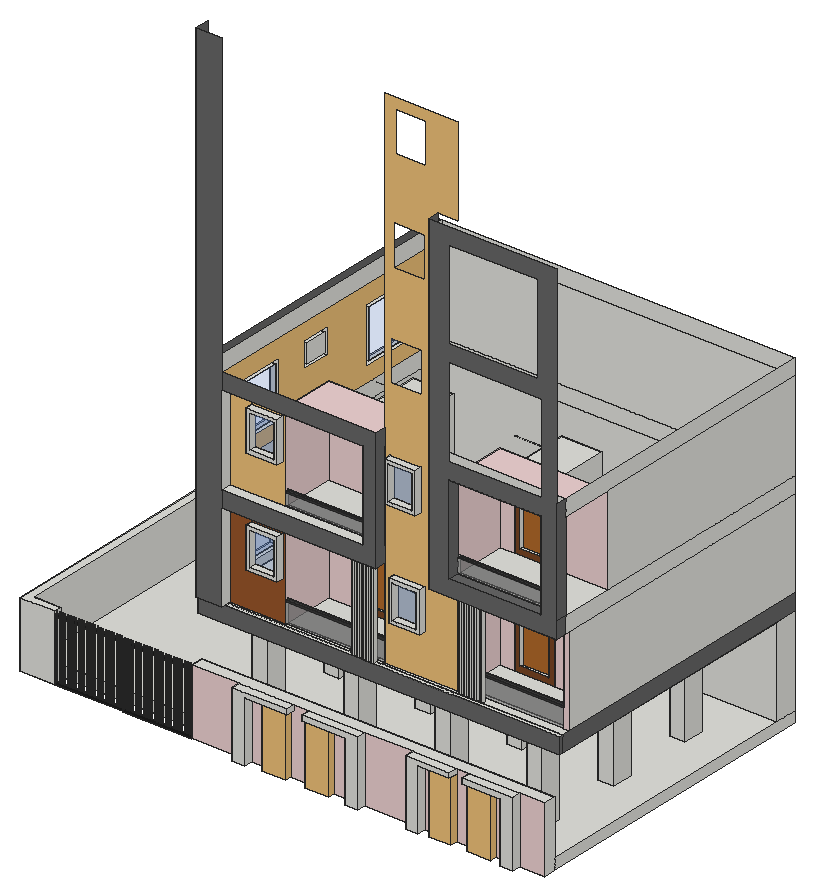
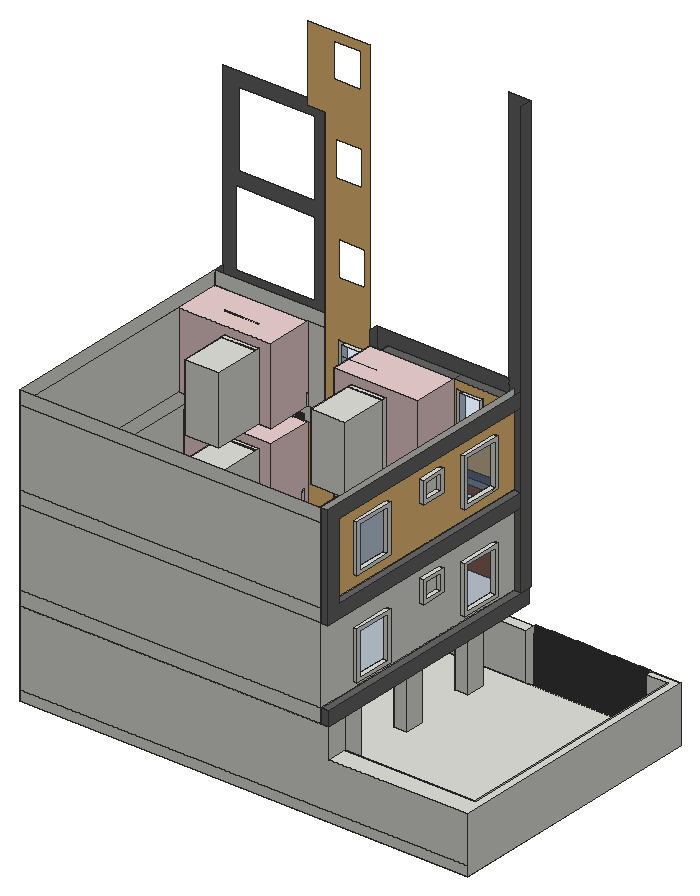
# SketchUp Ruby script. Lengths in inches.
U = 1.inch
M = Sketchup.active_model
def pt(a) = Geom::Point3d.new(a.map { |v| v * U })
def face(e, loops, mat)
  f = e.add_face(loops[0].map { |a| pt(a) })
  loops[1..].each { |l| e.add_face(l.map { |a| pt(a) }).erase! }
  f.material = f.back_material = mat if mat
  f
end
# faces: each face lists its corners as indices into pts; further lists are holes
def faces(e, pts, list, mat = nil) = list.each { |f| face(e, (f[0].is_a?(Array) ? f : [f]).map { |l| l.map { |i| pts[i] } }, mat) }
# xy, xz, yz: faces in a plane at the given z, y or x. An outline is a flat list of corners, or four numbers for a rectangle; further outlines are holes
def ring(l) = l.size == 4 ? [[l[0], l[1]], [l[2], l[1]], [l[2], l[3]], [l[0], l[3]]] : l.each_slice(2).to_a
def flat(e, list, mat, &to3) = list.each { |f| face(e, (f[0].is_a?(Array) ? f : [f]).map { |l| ring(l).map { |u, v| to3.(u, v) } }, mat) }
def xy(e, z, list, mat = nil) = flat(e, list, mat) { |x, y| [x, y, z] }
def xz(e, y, list, mat = nil) = flat(e, list, mat) { |x, z| [x, y, z] }
def yz(e, x, list, mat = nil) = flat(e, list, mat) { |y, z| [x, y, z] }
def lines(e, pts, list) = list.each { |a, b| e.add_line(pt(pts[a]), pt(pts[b])) }
# prism: a flat outline (further loops are holes) pulled along v
def prism(e, loops, v, mat = nil)
  f = face(e, loops, mat); d = Geom::Vector3d.new(v.map { |x| x * U })
  f.pushpull(f.normal.samedirection?(d) ? d.length : -d.length)
end
def box(e, o, s, mat = nil) = prism(e, [[o, [o[0] + s[0], o[1], o[2]], [o[0] + s[0], o[1] + s[1], o[2]], [o[0], o[1] + s[1], o[2]]]], [0, 0, s[2]], mat)
def at(x, y, z, deg = 0) = Geom::Transformation.translation(pt([x, y, z])) * Geom::Transformation.rotation(ORIGIN, Z_AXIS, deg.degrees)
def axes(o, x, y, z) = Geom::Transformation.new([*x, 0, *y, 0, *z, 0, *pt(o).to_a, 1])
def part(name) = M.definitions.add(name)
# library, detail: a bought-in or finely detailed component or shape, given as its bounding box
def library(name, o, s) = part(name).tap { |d| box(d.entities, o, s) }
def detail(e, o, s) = box(e.add_group.entities, o, s)
def put(e, d, t, mat = nil) = e.add_instance(d, t).tap { |i| i.material = mat if mat }
def group(e, t, mat = nil) = e.add_group.tap { |g| g.transformation = t; g.material = mat if mat }.entities
root = M.entities
M.materials.add("Generic").color = [103, 103, 103]
M.materials.add("Generic\#1").color = [239, 210, 210]
M.materials.add("[Color M07]").color = [58, 58, 58]
M.materials.add("[Color M08]").color = [30, 30, 30]
M.materials.add("[Translucent Glass Blue]").color = [98, 147, 234]
M.materials["[Translucent Glass Blue]"].alpha = 0.25
M.materials.add("[Translucent Glass Gray]").color = [128, 128, 128]
M.materials["[Translucent Glass Gray]"].alpha = 0.5
M.materials.add("[Wood Bamboo]").color = [177, 105, 43]
M.materials.add("[Wood Cherry Original]").color = [152, 86, 42]
M.materials.add("[Wood OSB]").color = [240, 195, 122]
M.materials.add("[Wood Veneer 01]").color = [120, 70, 37]
c1 = part("Group\#428")
prism(c1.entities,[[[0,1.97,0],[0,1.97,1.18],[0,0,1.18],[0,0,0]],[[0,1.92,1.13],[0,1.92,0.05],[0,0.05,0.05],[0,0.05,1.13]]],[98.43,0,0])
c2 = part("Group\#430")
xy(c2.entities,0,[[0.3,0,0.22,0.01,0.15,0.04,0.09,0.09,0.04,0.15,0.01,0.22,0,0.3,0.3,0.3],[0.3,0,0.3,0.3,0.59,0.3,0.58,0.22,0.55,0.15,0.5,0.09,0.44,0.04,0.37,0.01],[0,0.3,0.01,0.37,0.04,0.44,0.09,0.5,0.15,0.55,0.22,0.58,0.3,0.59,0.3,0.3],[0.3,0.3,0.3,0.59,0.37,0.58,0.44,0.55,0.5,0.5,0.55,0.44,0.58,0.37,0.59,0.3]])
xy(c2.entities,39.37,[[0.3,0,0.37,0.01,0.44,0.04,0.5,0.09,0.55,0.15,0.58,0.22,0.59,0.3,0.58,0.37,0.55,0.44,0.5,0.5,0.44,0.55,0.37,0.58,0.3,0.59,0.22,0.58,0.15,0.55,0.09,0.5,0.04,0.44,0.01,0.37,0,0.3,0.01,0.22,0.04,0.15,0.09,0.09,0.15,0.04,0.22,0.01]])
p = [[0.09,0.09,0],[0.15,0.04,0],[0.15,0.04,39.37],[0.09,0.09,39.37],[0.22,0.01,0],[0.22,0.01,39.37],
  [0.3,0,0],[0.3,0,39.37],[0.37,0.01,0],[0.37,0.01,39.37],[0.44,0.04,0],[0.44,0.04,39.37],
  [0.5,0.09,0],[0.5,0.09,39.37],[0.01,0.22,0],[0.04,0.15,0],[0.04,0.15,39.37],[0.01,0.22,39.37],
  [0.55,0.15,0],[0.55,0.15,39.37],[0.58,0.22,0],[0.58,0.22,39.37],[0,0.3,0],[0,0.3,39.37],
  [0.59,0.3,0],[0.59,0.3,39.37],[0.01,0.37,0],[0.01,0.37,39.37],[0.58,0.37,0],[0.58,0.37,39.37],
  [0.09,0.5,0],[0.04,0.44,0],[0.04,0.44,39.37],[0.09,0.5,39.37],[0.55,0.44,0],[0.5,0.5,0],
  [0.5,0.5,39.37],[0.55,0.44,39.37],[0.15,0.55,0],[0.15,0.55,39.37],[0.44,0.55,0],[0.44,0.55,39.37],
  [0.22,0.58,0],[0.22,0.58,39.37],[0.3,0.59,0],[0.3,0.59,39.37],[0.37,0.58,0],[0.37,0.58,39.37]]
faces(c2.entities,p,[[0,1,2,3],[1,4,5,2],[4,6,7,5],[6,8,9,7],[8,10,11,9],[10,12,13,11],[14,15,16,17],[15,0,3,16],
  [12,18,19,13],[18,20,21,19],[22,14,17,23],[20,24,25,21],[26,22,23,27],[24,28,29,25],[30,31,32,33],[31,26,27,32],
  [34,35,36,37],[28,34,37,29],[38,30,33,39],[35,40,41,36],[42,38,39,43],[44,42,43,45],[46,44,45,47],[40,46,47,41]])
c3 = part("Group\#429")
prism(c3.entities,[[[0.01,0.22,35.83],[0,0.3,35.83],[0.01,0.37,35.83],[0.04,0.44,35.83],[0.09,0.5,35.83],[0.15,0.55,35.83],[0.22,0.58,35.83],[0.3,0.59,35.83],[0.37,0.58,35.83],[0.44,0.55,35.83],[0.5,0.5,35.83],[0.55,0.44,35.83],[0.58,0.37,35.83],[0.59,0.3,35.83],[0.58,0.22,35.83],[0.55,0.15,35.83],[0.5,0.09,35.83],[0.44,0.04,35.83],[0.37,0.01,35.83],[0.3,0,35.83],[0.22,0.01,35.83],[0.15,0.04,35.83],[0.09,0.09,35.83],[0.04,0.15,35.83]]],[0,0,3.54])
c4 = part("Barred gate panel")
g1 = group(c4.entities,at(0,0,0))
put(g1,c1,axes([0,0,39.76],[1,0,0],[0,0,-1],[0,1,0]),"[Color M08]")
put(g1,c1,axes([0,0,1.97],[1,0,0],[0,0,-1],[0,1,0]),"[Color M08]")
put(g1,c1,axes([98.43,0,37.8],[0,0,-0.364],[-1,0,0],[0,1,0]),"[Color M08]")
put(g1,c1,axes([1.97,0,37.8],[0,0,-0.364],[-1,0,0],[0,1,0]),"[Color M08]")
g2 = group(c4.entities,at(1.67,0.3,1.97))
put(g2,c2,at(78.74,0,0),"[Color M08]")
put(g2,c2,at(90.55,0,0),"[Color M08]")
put(g2,c2,at(82.68,0,0),"[Color M08]")
put(g2,c2,at(86.61,0,0),"[Color M08]")
put(g2,c2,at(66.93,0,0),"[Color M08]")
put(g2,c2,at(11.8125,0,0),"[Color M08]")
put(g2,c2,at(15.75,0,0),"[Color M08]")
put(g2,c2,at(47.24,0,0),"[Color M08]")
put(g2,c2,at(59.06,0,0),"[Color M08]")
put(g2,c3,at(0,0,0),"[Color M08]")
put(g2,c2,at(39.37,0,0),"[Color M08]")
put(g2,c2,at(62.99,0,0),"[Color M08]")
put(g2,c2,at(55.12,0,0),"[Color M08]")
put(g2,c2,at(19.69,0,0),"[Color M08]")
put(g2,c2,at(35.43,0,0),"[Color M08]")
put(g2,c2,at(7.875,0,0),"[Color M08]")
put(g2,c2,at(23.62,0,0),"[Color M08]")
put(g2,c2,at(31.5,0,0),"[Color M08]")
put(g2,c2,at(43.31,0,0),"[Color M08]")
put(g2,c2,at(27.56,0,0),"[Color M08]")
put(g2,c2,at(3.9375,0,0),"[Color M08]")
put(g2,c2,at(51.18,0,0),"[Color M08]")
put(g2,c2,at(70.87,0,0),"[Color M08]")
put(g2,c2,at(74.8,0,0),"[Color M08]")
put(g2,c3,at(94.49,0,0),"[Color M08]")
c5 = part("Group\#1")
xy(c5.entities,0,[[0,0,76.25,8.9375]])
xy(c5.entities,11.01,[[11.01,0,65.24,5.9375]])
xy(c5.entities,138.8,[[11.01,0,65.24,5.9375]])
xy(c5.entities,149.8125,[[0,0,76.25,8.9375]])
xz(c5.entities,0,[[[0,0,76.25,149.8125],[11.01,11.01,65.24,138.8]]],"[Wood Veneer 01]")
xz(c5.entities,5.9375,[[11.01,11.01,65.24,138.8]],"[Wood Bamboo]")
xz(c5.entities,8.9375,[[0,0,76.25,149.8125]])
yz(c5.entities,0,[[0,0,8.9375,149.8125]])
yz(c5.entities,11.01,[[0,11.01,5.9375,138.8]])
yz(c5.entities,65.24,[[0,11.01,5.9375,138.8]])
yz(c5.entities,76.25,[[0,0,8.9375,149.8125]])
xy(root,-20.9375,[[412.81,0,412.81,16.75,323.875,16.75,323.875,40.1875,989.0625,40.1875,989.0625,16.75,942.13,16.75,942.13,0,918.69,0,918.69,16.75,897.59,16.75,897.59,4.0625,852.34,4.0625,852.34,16.75,822.94,16.75,822.94,4.0625,780.96,4.0625,780.96,16.75,763.51,16.75,763.51,0,740.07,0,740.07,16.75,650.38,16.75,650.38,0,625.95,0,625.95,16.75,592.21,16.75,592.21,4.0625,546.96,4.0625,546.96,16.75,510.84,16.75,510.84,4.0625,465.59,4.0625,465.59,16.75,437.72,16.75,437.72,0],[0,16.75,0,606.43,989.0625,606.43,989.0625,40.1875,16.9375,40.1875,16.9375,30.9375,66.25,30.9375,66.25,16.75]])
xy(root,0,[[[16.9375,40.1875,989.0625,563.74],[375.33,94.8,404.7,134.68],[547.72,94.8,577.1,134.68],[720.12,94.8,749.49,134.68],[892.51,94.8,921.89,134.68],[892.51,263.49,921.89,303.36],[720.12,263.49,749.49,303.36],[547.72,263.49,577.1,303.36],[375.33,263.49,404.7,303.36],[892.51,432.18,921.89,472.05],[720.12,432.18,749.49,472.05],[547.72,432.18,577.1,472.05],[375.33,432.18,404.7,472.05]]])
xy(root,92.29,[[544.32,0,544.32,16.75,546.96,16.75,546.96,4.0625,592.21,4.0625,592.21,16.75,625.95,16.75,625.95,0],[546.96,4.0625,592.21,16.75],[780.96,4.0625,822.94,16.75],[852.34,4.0625,897.59,16.75]])
xy(root,92.62,[[846.69,0,918.69,16.75]])
xy(root,93.7,[[437.72,0,437.72,16.75,465.59,16.75,465.59,4.0625,510.84,4.0625,510.84,16.75,517.1,16.75,517.1,0]])
xy(root,93.72,[[763.51,0,822.94,16.75]])
xy(root,102.9375,[[412.81,0,517.1,16.75],[544.32,0,650.38,16.75],[740.07,0,822.94,16.75],[846.69,0,942.13,16.75],[0,16.75,66.25,16.75,66.25,30.9375,16.9375,30.9375,16.9375,563.74,305.5625,563.74,305.5625,606.43,0,606.43],
  [323.875,16.75,989.0625,40.1875]])
xy(root,164.6875,[[375.33,94.8,404.7,134.68],[547.72,94.8,577.1,134.68],[720.12,94.8,749.49,134.68],[892.51,94.8,921.89,134.68],[375.33,263.49,404.7,303.36],
  [547.72,263.49,577.1,303.36],[720.12,263.49,749.49,303.36],[892.51,263.49,921.89,303.36],[375.33,432.18,404.7,472.05],[547.72,432.18,577.1,472.05],
  [720.12,432.18,749.49,472.05],[892.51,432.18,921.89,472.05]])
xy(root,168,[[323.875,61.13,989.0625,563.74],[323.875,563.74,989.0625,606.43]])
xy(root,168,[[305.5625,53.875,305.5625,563.74,323.875,563.74,323.875,61.13,989.0625,61.13,989.0625,53.875],[305.5625,563.74,323.875,606.43]],"Generic")
xy(root,198.625,[[307.875,53.875,356.25,61.13],[356.25,53.875,461.64,61.13],[461.64,53.875,596.35,61.13],[596.35,53.875,601.6,61.13],[601.6,53.875,605.17,61.13],
  [605.17,53.875,610.42,61.13],[610.42,53.875,613.98,61.13],[613.98,53.875,619.23,61.13],[619.23,53.875,622.79,61.13],[622.79,53.875,628.04,61.13],
  [628.04,53.875,631.6,61.13],[631.6,53.875,636.85,61.13],[636.85,53.875,647.41,61.13],[647.41,53.875,785.17,61.13],[785.17,53.875,792.52,61.13],
  [792.52,53.875,797.96,61.13],[797.96,53.875,802.08,61.13],[802.08,53.875,807.52,61.13],[807.52,53.875,811.64,61.13],[811.64,53.875,817.08,61.13],
  [817.08,53.875,821.21,61.13],[821.21,53.875,826.64,61.13],[826.64,53.875,830.77,61.13],[830.77,53.875,836.21,61.13],[836.21,53.875,989.0625,61.13],
  [307.875,61.13,323.875,73.93],[323.875,61.13,323.875,606.43,989.0625,606.43,989.0625,76.18,978.875,76.18,978.875,167.12,888.25,167.12,888.25,277.93,812,277.93,812,167.12,785.17,167.12,785.17,66.43,647.41,66.43,647.41,167.12,603.16,167.12,603.16,277.93,526.91,277.93,526.91,167.12,461.64,167.12,461.64,66.43,356.25,66.43,356.25,61.13],[356.25,61.13,461.64,66.43],[461.64,61.13,596.35,61.13,596.35,62.37,601.6,62.37,601.6,61.13,605.17,61.13,605.17,62.37,610.42,62.37,610.42,61.13,613.98,61.13,613.98,62.37,619.23,62.37,619.23,61.13,622.79,61.13,622.79,62.37,628.04,62.37,628.04,61.13,631.6,61.13,631.6,62.37,636.85,62.37,636.85,61.13,647.41,61.13,647.41,66.43,461.64,66.43],[647.41,61.13,785.17,66.43],
  [785.17,61.13,785.17,76.18,989.0625,76.18,989.0625,61.13,836.21,61.13,836.21,66.56,830.77,66.56,830.77,61.13,826.64,61.13,826.64,66.56,821.21,66.56,821.21,61.13,817.08,61.13,817.08,66.56,811.64,66.56,811.64,61.13,807.52,61.13,807.52,66.56,802.08,66.56,802.08,61.13,797.96,61.13,797.96,66.56,792.52,66.56,792.52,61.13],[792.52,61.13,797.96,66.56],[802.08,61.13,807.52,66.56],[811.64,61.13,817.08,66.56],[821.21,61.13,826.64,66.56],
  [830.77,61.13,836.21,66.56],[461.64,66.43,647.41,72.12],[461.64,72.12,461.64,167.12,526.91,167.12,526.91,277.93,603.16,277.93,603.16,167.12,647.41,167.12,647.41,72.12],[785.17,76.18,978.875,83.18],[785.17,83.18,785.17,167.12,812,167.12,812,277.93,888.25,277.93,888.25,167.12,978.875,167.12,978.875,83.18]])
xy(root,198.625,[[307.875,45.93,356.25,53.875],[305.5625,53.875,307.875,53.875,307.875,73.93,323.875,73.93,323.875,606.43,305.5625,606.43]],"Generic")
xy(root,213.74,[[313.8125,129.65,323.875,221.17],[313.8125,426.9,323.875,518.42]])
xy(root,220.56,[[313.8125,136.47,323.875,214.35],[313.8125,433.72,323.875,511.6]])
xy(root,233.5625,[[785.17,76.18,978.875,83.18]])
xy(root,235,[[461.64,66.43,647.41,72.12]])
xy(root,237,[[785.17,76.18,978.875,83.18]],"[Color M07]")
xy(root,239.625,[[461.64,66.43,647.41,72.12]],"[Color M07]")
xy(root,272.41,[[397.09,53.18,455.09,66.43]])
xy(root,277.45,[[666.1,53.18,724.1,66.43]])
xy(root,278.91,[[403.59,53.18,448.59,66.43]])
xy(root,283.95,[[672.6,53.18,717.6,66.43]])
xy(root,288.87,[[312.6875,281.29,323.875,336.99]])
xy(root,295.6875,[[312.6875,288.11,323.875,330.17]])
xy(root,312.56,[[313.8125,136.47,323.875,214.35],[313.8125,433.72,323.875,511.6]])
xy(root,319.375,[[313.8125,129.65,323.875,221.17],[313.8125,426.9,323.875,518.42]])
xy(root,330.375,[[312.6875,288.11,323.875,330.17]])
xy(root,337.2,[[312.6875,281.29,323.875,336.99]])
xy(root,342.54,[[403.59,53.18,448.59,66.43]])
xy(root,347.4375,[[526.91,167.12,603.16,277.93],[812,167.12,888.25,277.93]])
xy(root,347.58,[[672.6,53.18,717.6,66.43]])
xy(root,349.04,[[397.09,53.18,455.09,66.43]])
xy(root,354.08,[[666.1,53.18,724.1,66.43]])
xy(root,366.625,[[356.25,45.93,647.41,66.43],[748.05,45.93,989.0625,66.43],[307.875,73.93,323.875,606.43]],"Generic")
xy(root,366.625,[[461.64,66.43,647.41,167.12],[785.17,66.43,785.17,167.12,978.875,167.12,978.875,76.18,989.0625,76.18,989.0625,66.43]],"Generic\#1")
xy(root,372.25,[[821.21,61.13,826.64,66.56],[830.77,61.13,836.21,66.56]])
xy(root,379.9375,[[792.52,61.13,797.96,66.56],[802.08,61.13,807.52,66.56],[811.64,61.13,817.08,66.56]])
xy(root,382.0625,[[596.35,53.875,601.6,62.37],[605.17,53.875,610.42,62.37],[613.98,53.875,619.23,62.37],[622.79,53.875,628.04,62.37],[631.6,53.875,636.85,62.37]])
xy(root,397.25,[[356.25,45.93,623.41,66.43],[461.64,66.43,623.41,71.31],[623.41,66.43,623.41,71.31,461.64,71.31,461.64,167.12,532.74,167.12,532.74,277.93,608.99,277.93,608.99,167.12,647.41,167.12,647.41,66.43],[785.17,66.43,958.0625,70.99],[958.0625,66.43,958.0625,70.99,785.17,70.99,785.17,167.12,812,167.12,812,277.93,888.25,277.93,888.25,167.12,989.0625,167.12,989.0625,66.43]])
xy(root,397.25,[[785.17,45.93,958.0625,66.43],[307.875,73.93,323.875,577.37]],"Generic")
xy(root,420.375,[[461.64,66.43,623.41,71.31]])
xy(root,423.6875,[[785.17,66.43,958.0625,70.99]])
xy(root,423.8125,[[461.64,66.43,623.41,71.31]],"[Color M07]")
xy(root,425.86,[[313.8125,129.65,323.875,221.17],[313.8125,426.9,323.875,518.42]])
xy(root,426.0625,[[785.17,66.43,958.0625,70.99]],"[Color M07]")
xy(root,432.68,[[313.8125,136.47,323.875,214.35],[313.8125,433.72,323.875,511.6]])
xy(root,470.79,[[397.09,53.18,455.09,66.43]])
xy(root,475.87,[[658.08,53.18,716.08,66.43]])
xy(root,477.29,[[403.59,53.18,448.59,66.43]])
xy(root,482.375,[[664.58,53.18,709.58,66.43]])
xy(root,486.06,[[312.6875,281.29,323.875,336.99]])
xy(root,492.875,[[312.6875,288.11,323.875,330.17]])
xy(root,524.68,[[313.8125,136.47,323.875,214.35],[313.8125,433.72,323.875,511.6]])
xy(root,527.5625,[[312.6875,288.11,323.875,330.17]])
xy(root,531.5,[[313.8125,129.65,323.875,221.17],[313.8125,426.9,323.875,518.42]])
xy(root,534.38,[[312.6875,281.29,323.875,336.99]])
xy(root,540.91,[[403.59,53.18,448.59,66.43]])
xy(root,546,[[664.58,53.18,709.58,66.43]])
xy(root,546.0625,[[532.74,167.12,608.99,277.93],[812,167.12,888.25,277.93]])
xy(root,547.42,[[397.09,53.18,455.09,66.43]])
xy(root,552.5,[[658.08,53.18,716.08,66.43]])
xy(root,565.25,[[356.25,45.93,461.64,66.43],[461.64,45.93,623.41,66.43],[785.17,45.93,958.0625,66.43],[307.875,73.93,323.875,577.37]],"Generic")
xy(root,565.25,[[461.64,66.43,647.41,167.12],[785.17,66.43,989.0625,167.12]],"Generic\#1")
xz(root,0,[[412.81,-20.9375,437.72,-20.9375,437.72,93.7,517.1,93.7,517.1,102.9375,412.81,102.9375],[625.95,-20.9375,650.38,-20.9375,650.38,102.9375,544.32,102.9375,544.32,92.29,625.95,92.29],[740.07,-20.9375,763.51,-20.9375,763.51,93.72,822.94,93.72,822.94,102.9375,740.07,102.9375],[918.69,-20.9375,942.13,-20.9375,942.13,102.9375,846.69,102.9375,846.69,92.62,918.69,92.62]])
xz(root,4.0625,[[465.59,-20.9375,510.84,93.7],[546.96,-20.9375,592.21,92.29],[780.96,-20.9375,822.94,92.29],[852.34,-20.9375,897.59,92.29]],"[Wood OSB]")
xz(root,16.75,[[0,-20.9375,66.25,102.9375],[546.96,92.29,592.21,93.7],[852.34,92.29,897.59,92.62]])
xz(root,16.75,[[323.875,-20.9375,412.81,102.9375],[437.72,-20.9375,465.59,93.7],[510.84,-20.9375,546.96,-20.9375,546.96,92.29,544.32,92.29,544.32,102.9375,517.1,102.9375,517.1,93.7,510.84,93.7],[592.21,-20.9375,625.95,92.29],[650.38,-20.9375,740.07,102.9375],
  [763.51,-20.9375,780.96,-20.9375,780.96,92.29,822.94,92.29,822.94,-20.9375,852.34,-20.9375,852.34,92.62,846.69,92.62,846.69,102.9375,822.94,102.9375,822.94,93.72,763.51,93.72],[897.59,-20.9375,918.69,92.62],[942.13,-20.9375,989.0625,102.9375]],"Generic\#1")
xz(root,30.9375,[[16.9375,-20.9375,66.25,102.9375]])
xz(root,40.1875,[[16.9375,-20.9375,323.875,0],[323.875,-20.9375,989.0625,0],[323.875,0,989.0625,102.9375]])
xz(root,45.93,[[307.875,198.625,356.25,1161.125],[356.25,366.625,647.41,366.625,647.41,595.875,356.25,595.875,356.25,565.25,623.41,565.25,623.41,397.25,356.25,397.25],[[748.05,366.625,989.0625,993.125],[785.17,595.875,960.48,763.875],[785.17,397.25,958.0625,565.25],[785.17,794.5,952.9375,962.5]]],"Generic")
xz(root,53.18,[[[397.09,272.41,455.09,349.04],[403.59,278.91,448.59,342.54]],[[666.1,277.45,724.1,354.08],[672.6,283.95,717.6,347.58]],[[397.09,470.79,455.09,547.42],[403.59,477.29,448.59,540.91]],[[658.08,475.87,716.08,552.5],[664.58,482.375,709.58,546]]])
xz(root,53.875,[[596.35,198.625,601.6,382.0625],[605.17,198.625,610.42,382.0625],[613.98,198.625,619.23,382.0625],[622.79,198.625,628.04,382.0625],[631.6,198.625,636.85,382.0625]])
xz(root,53.875,[[305.5625,168,989.0625,198.625]],"Generic")
xz(root,61.13,[[323.875,168,989.0625,198.625],[792.52,198.625,797.96,379.9375],[802.08,198.625,807.52,379.9375],[811.64,198.625,817.08,379.9375],[821.21,198.625,826.64,372.25],
  [830.77,198.625,836.21,372.25]])
xz(root,62.37,[[596.35,198.625,601.6,382.0625],[605.17,198.625,610.42,382.0625],[613.98,198.625,619.23,382.0625],[622.79,198.625,628.04,382.0625],[631.6,198.625,636.85,382.0625]])
xz(root,66.43,[[748.05,366.625,989.0625,397.25],[623.41,397.25,647.41,565.25],[748.05,397.25,785.17,565.25],[958.0625,397.25,989.0625,565.25],[748.05,565.25,989.0625,595.875]])
xz(root,66.43,[[461.64,235,647.41,239.625],[461.64,420.375,623.41,423.8125],[785.17,423.6875,958.0625,426.0625]],"[Color M07]")
xz(root,66.43,[[403.59,278.91,448.59,342.54],[672.6,283.95,717.6,347.58],[403.59,477.29,448.59,540.91],[664.58,482.375,709.58,546]],"[Translucent Glass Blue]")
xz(root,66.43,[[461.64,198.625,647.41,235],[461.64,397.25,623.41,420.375],[785.17,397.25,958.0625,423.6875]],"[Translucent Glass Gray]")
xz(root,66.43,[[[356.25,198.625,461.64,366.625],[397.09,272.41,455.09,349.04]]],"[Wood Cherry Original]")
xz(root,66.43,[[[647.41,198.625,785.17,198.625,785.17,366.625,748.05,366.625,748.05,993.125,785.17,993.125,785.17,1161.125,647.41,1161.125],[666.1,277.45,724.1,354.08],[659.17,675.14,717.17,751.77],[664.84,871.85,722.84,948.48],[668.28,1064.99,726.28,1141.625],[658.08,475.87,716.08,552.5]],[[356.25,397.25,461.64,565.25],[397.09,470.79,455.09,547.42]]],"[Wood OSB]")
xz(root,66.56,[[792.52,198.625,797.96,379.9375],[802.08,198.625,807.52,379.9375],[811.64,198.625,817.08,379.9375],[821.21,198.625,826.64,372.25],[830.77,198.625,836.21,372.25]])
xz(root,70.99,[[785.17,423.6875,958.0625,426.0625]])
xz(root,70.99,[[785.17,397.25,958.0625,423.6875]],"[Translucent Glass Gray]")
xz(root,71.31,[[461.64,420.375,623.41,423.8125]])
xz(root,71.31,[[461.64,397.25,623.41,420.375]],"[Translucent Glass Gray]")
xz(root,72.12,[[461.64,235,647.41,239.625]])
xz(root,72.12,[[461.64,198.625,647.41,235]],"[Translucent Glass Gray]")
xz(root,73.93,[[307.875,198.625,323.875,366.625],[307.875,397.25,323.875,565.25]],"Generic")
xz(root,76.18,[[978.875,198.625,989.0625,366.625]],"Generic\#1")
xz(root,76.18,[[785.17,233.5625,978.875,237]],"[Color M07]")
xz(root,76.18,[[785.17,198.625,978.875,233.5625]],"[Translucent Glass Gray]")
xz(root,83.18,[[785.17,233.5625,978.875,237]])
xz(root,83.18,[[785.17,198.625,978.875,233.5625]],"[Translucent Glass Gray]")
xz(root,94.8,[[375.33,0,404.7,164.6875],[547.72,0,577.1,164.6875],[720.12,0,749.49,164.6875],[892.51,0,921.89,164.6875]])
xz(root,129.65,[[313.8125,213.74,323.875,319.375],[313.8125,425.86,323.875,531.5]])
xz(root,134.68,[[375.33,0,404.7,164.6875],[547.72,0,577.1,164.6875],[720.12,0,749.49,164.6875],[892.51,0,921.89,164.6875]])
xz(root,136.47,[[313.8125,220.56,323.875,312.56],[313.8125,432.68,323.875,524.68]])
xz(root,167.12,[[812,594.875,888.25,595.875]])
xz(root,167.12,[[461.64,198.625,526.91,198.625,526.91,347.4375,603.16,347.4375,603.16,198.625,647.41,198.625,647.41,366.625,461.64,366.625],[785.17,198.625,812,198.625,812,347.4375,888.25,347.4375,888.25,198.625,978.875,198.625,978.875,366.625,785.17,366.625],[461.64,397.25,532.74,397.25,532.74,546.0625,608.99,546.0625,608.99,397.25,647.41,397.25,647.41,565.25,461.64,565.25],[785.17,397.25,812,397.25,812,546.0625,888.25,546.0625,888.25,397.25,989.0625,397.25,989.0625,565.25,785.17,565.25]],"Generic\#1")
xz(root,214.35,[[313.8125,220.56,323.875,312.56],[313.8125,432.68,323.875,524.68]])
xz(root,221.17,[[313.8125,213.74,323.875,319.375],[313.8125,425.86,323.875,531.5]])
xz(root,263.49,[[375.33,0,404.7,164.6875],[547.72,0,577.1,164.6875],[720.12,0,749.49,164.6875],[892.51,0,921.89,164.6875]])
xz(root,277.93,[[526.91,198.625,603.16,347.4375],[812,198.625,888.25,347.4375],[532.74,397.25,608.99,546.0625],[812,397.25,888.25,546.0625]])
xz(root,281.29,[[312.6875,288.87,323.875,337.2],[312.6875,486.06,323.875,534.38]])
xz(root,288.11,[[312.6875,295.6875,323.875,330.375],[312.6875,492.875,323.875,527.5625]])
xz(root,303.36,[[375.33,0,404.7,164.6875],[547.72,0,577.1,164.6875],[720.12,0,749.49,164.6875],[892.51,0,921.89,164.6875]])
xz(root,330.17,[[312.6875,295.6875,323.875,330.375],[312.6875,492.875,323.875,527.5625]])
xz(root,336.99,[[312.6875,288.87,323.875,337.2],[312.6875,486.06,323.875,534.38]])
xz(root,426.9,[[313.8125,213.74,323.875,319.375],[313.8125,425.86,323.875,531.5]])
xz(root,432.18,[[375.33,0,404.7,164.6875],[547.72,0,577.1,164.6875],[720.12,0,749.49,164.6875],[892.51,0,921.89,164.6875]])
xz(root,433.72,[[313.8125,220.56,323.875,312.56],[313.8125,432.68,323.875,524.68]])
xz(root,472.05,[[375.33,0,404.7,164.6875],[547.72,0,577.1,164.6875],[720.12,0,749.49,164.6875],[892.51,0,921.89,164.6875]])
xz(root,511.6,[[313.8125,220.56,323.875,312.56],[313.8125,432.68,323.875,524.68]])
xz(root,518.42,[[313.8125,213.74,323.875,319.375],[313.8125,425.86,323.875,531.5]])
xz(root,563.74,[[16.9375,0,989.0625,0,989.0625,168,305.5625,168,305.5625,102.9375,16.9375,102.9375]])
xz(root,577.37,[[307.875,397.25,323.875,565.25]],"Generic")
xz(root,606.43,[[0,-20.9375,989.0625,0],[0,0,0,102.9375,305.5625,102.9375,305.5625,168,989.0625,168,989.0625,0],[323.875,168,989.0625,198.625],[323.875,198.625,989.0625,366.625],[323.875,366.625,989.0625,397.25],
  [323.875,397.25,989.0625,565.25],[323.875,565.25,989.0625,595.875]])
xz(root,606.43,[[305.5625,168,323.875,198.625],[307.875,366.625,323.875,595.875]],"Generic")
yz(root,0,[[16.75,-20.9375,606.43,102.9375]])
yz(root,16.9375,[[30.9375,-20.9375,40.1875,-20.9375,40.1875,0,563.74,0,563.74,102.9375,30.9375,102.9375]])
yz(root,66.25,[[16.75,-20.9375,30.9375,102.9375]])
yz(root,305.5625,[[563.74,102.9375,606.43,168]])
yz(root,305.5625,[[53.875,168,606.43,198.625]],"Generic")
yz(root,307.875,[[45.93,198.625,73.93,1161.125],[73.93,366.625,73.93,397.25,577.37,397.25,577.37,565.25,73.93,565.25,73.93,595.875,606.43,595.875,606.43,366.625]],"Generic")
yz(root,312.6875,[[[281.29,288.87,336.99,337.2],[288.11,295.6875,330.17,330.375]],[[281.29,486.06,336.99,534.38],[288.11,492.875,330.17,527.5625]]])
yz(root,313.8125,[[[129.65,213.74,221.17,319.375],[136.47,220.56,214.35,312.56]],[[426.9,213.74,518.42,319.375],[433.72,220.56,511.6,312.56]],[[129.65,425.86,221.17,531.5],[136.47,432.68,214.35,524.68]],[[426.9,425.86,518.42,531.5],[433.72,432.68,511.6,524.68]]])
yz(root,323.875,[[16.75,-20.9375,40.1875,102.9375],[61.13,168,606.43,198.625],[[73.93,198.625,606.43,366.625],[129.65,213.74,221.17,319.375],[426.9,213.74,518.42,319.375],[281.29,288.87,336.99,337.2]],[288.11,295.6875,330.17,330.375],[73.93,366.625,73.93,397.25,577.37,397.25,577.37,565.25,73.93,565.25,73.93,595.875,606.43,595.875,606.43,366.625],
  [288.11,492.875,330.17,527.5625]])
yz(root,323.875,[[136.47,220.56,214.35,312.56],[433.72,220.56,511.6,312.56],[136.47,432.68,214.35,524.68],[433.72,432.68,511.6,524.68]],"[Translucent Glass Blue]")
yz(root,323.875,[[[73.93,397.25,577.37,565.25],[129.65,425.86,221.17,531.5],[426.9,425.86,518.42,531.5],[281.29,486.06,336.99,534.38]]],"[Wood OSB]")
yz(root,356.25,[[45.93,198.625,66.43,366.625],[45.93,397.25,66.43,565.25]])
yz(root,375.33,[[94.8,0,134.68,164.6875],[263.49,0,303.36,164.6875],[432.18,0,472.05,164.6875]])
yz(root,397.09,[[53.18,272.41,66.43,349.04],[53.18,470.79,66.43,547.42]])
yz(root,403.59,[[53.18,278.91,66.43,342.54],[53.18,477.29,66.43,540.91]])
yz(root,404.7,[[94.8,0,134.68,164.6875],[263.49,0,303.36,164.6875],[432.18,0,472.05,164.6875]])
yz(root,412.81,[[0,-20.9375,16.75,102.9375]])
yz(root,437.72,[[0,-20.9375,16.75,93.7]])
yz(root,448.59,[[53.18,278.91,66.43,342.54],[53.18,477.29,66.43,540.91]])
yz(root,455.09,[[53.18,272.41,66.43,349.04],[53.18,470.79,66.43,547.42]])
yz(root,461.64,[[66.43,198.625,72.12,235],[66.43,235,72.12,239.625],[66.43,397.25,71.31,420.375],[66.43,420.375,71.31,423.8125]])
yz(root,461.64,[[72.12,198.625,167.12,198.625,167.12,366.625,66.43,366.625,66.43,239.625,72.12,239.625],[71.31,397.25,167.12,397.25,167.12,565.25,66.43,565.25,66.43,423.8125,71.31,423.8125]],"Generic\#1")
yz(root,465.59,[[4.0625,-20.9375,16.75,93.7]],"[Wood OSB]")
yz(root,510.84,[[4.0625,-20.9375,16.75,93.7]],"[Wood OSB]")
yz(root,517.1,[[0,93.7,16.75,102.9375]])
yz(root,526.91,[[167.12,198.625,277.93,347.4375]])
yz(root,532.74,[[167.12,397.25,277.93,546.0625]])
yz(root,544.32,[[0,92.29,16.75,102.9375]])
yz(root,546.96,[[4.0625,-20.9375,16.75,92.29]],"[Wood OSB]")
yz(root,547.72,[[94.8,0,134.68,164.6875],[263.49,0,303.36,164.6875],[432.18,0,472.05,164.6875]])
yz(root,577.1,[[94.8,0,134.68,164.6875],[263.49,0,303.36,164.6875],[432.18,0,472.05,164.6875]])
yz(root,592.21,[[4.0625,-20.9375,16.75,92.29]],"[Wood OSB]")
yz(root,596.35,[[53.875,198.625,62.37,382.0625]])
yz(root,601.6,[[53.875,198.625,62.37,382.0625]])
yz(root,603.16,[[167.12,198.625,277.93,347.4375]])
yz(root,605.17,[[53.875,198.625,62.37,382.0625]])
yz(root,608.99,[[167.12,397.25,277.93,546.0625]])
yz(root,610.42,[[53.875,198.625,62.37,382.0625]])
yz(root,613.98,[[53.875,198.625,62.37,382.0625]])
yz(root,619.23,[[53.875,198.625,62.37,382.0625]])
yz(root,622.79,[[53.875,198.625,62.37,382.0625]])
yz(root,623.41,[[66.43,397.25,71.31,420.375],[66.43,420.375,71.31,423.8125]])
yz(root,623.41,[[45.93,397.25,66.43,565.25]],"Generic")
yz(root,625.95,[[0,-20.9375,16.75,92.29]])
yz(root,628.04,[[53.875,198.625,62.37,382.0625]])
yz(root,631.6,[[53.875,198.625,62.37,382.0625]])
yz(root,636.85,[[53.875,198.625,62.37,382.0625]])
yz(root,647.41,[[66.43,198.625,72.12,235],[72.12,198.625,72.12,239.625,66.43,239.625,66.43,366.625,167.12,366.625,167.12,198.625],[66.43,235,72.12,239.625],[66.43,397.25,167.12,565.25]])
yz(root,647.41,[[45.93,366.625,66.43,595.875]],"Generic")
yz(root,650.38,[[0,-20.9375,16.75,102.9375]])
yz(root,658.08,[[53.18,475.87,66.43,552.5]])
yz(root,664.58,[[53.18,482.375,66.43,546]])
yz(root,666.1,[[53.18,277.45,66.43,354.08]])
yz(root,672.6,[[53.18,283.95,66.43,347.58]])
yz(root,709.58,[[53.18,482.375,66.43,546]])
yz(root,716.08,[[53.18,475.87,66.43,552.5]])
yz(root,717.6,[[53.18,283.95,66.43,347.58]])
yz(root,720.12,[[94.8,0,134.68,164.6875],[263.49,0,303.36,164.6875],[432.18,0,472.05,164.6875]])
yz(root,724.1,[[53.18,277.45,66.43,354.08]])
yz(root,740.07,[[0,-20.9375,16.75,102.9375]])
yz(root,748.05,[[45.93,366.625,66.43,993.125]],"Generic")
yz(root,749.49,[[94.8,0,134.68,164.6875],[263.49,0,303.36,164.6875],[432.18,0,472.05,164.6875]])
yz(root,763.51,[[0,-20.9375,16.75,93.72]])
yz(root,780.96,[[4.0625,-20.9375,16.75,92.29]],"[Wood OSB]")
yz(root,785.17,[[76.18,198.625,83.18,233.5625],[76.18,233.5625,83.18,237],[66.43,397.25,70.99,423.6875],[66.43,423.6875,70.99,426.0625]])
yz(root,785.17,[[45.93,397.25,66.43,565.25]],"Generic")
yz(root,785.17,[[66.43,198.625,76.18,198.625,76.18,237,83.18,237,83.18,198.625,167.12,198.625,167.12,366.625,66.43,366.625],[70.99,397.25,167.12,397.25,167.12,565.25,66.43,565.25,66.43,426.0625,70.99,426.0625]],"Generic\#1")
yz(root,792.52,[[61.13,198.625,66.56,379.9375]])
yz(root,797.96,[[61.13,198.625,66.56,379.9375]])
yz(root,802.08,[[61.13,198.625,66.56,379.9375]])
yz(root,807.52,[[61.13,198.625,66.56,379.9375]])
yz(root,811.64,[[61.13,198.625,66.56,379.9375]])
yz(root,812,[[167.12,198.625,277.93,347.4375],[167.12,397.25,277.93,546.0625]])
yz(root,817.08,[[61.13,198.625,66.56,379.9375]])
yz(root,821.21,[[61.13,198.625,66.56,372.25]])
yz(root,822.94,[[0,93.72,16.75,102.9375]])
yz(root,822.94,[[4.0625,-20.9375,16.75,92.29]],"[Wood OSB]")
yz(root,826.64,[[61.13,198.625,66.56,372.25]])
yz(root,830.77,[[61.13,198.625,66.56,372.25]])
yz(root,836.21,[[61.13,198.625,66.56,372.25]])
yz(root,846.69,[[0,92.62,16.75,102.9375]])
yz(root,852.34,[[4.0625,-20.9375,16.75,92.29]],"[Wood OSB]")
yz(root,888.25,[[167.12,198.625,277.93,347.4375],[167.12,397.25,277.93,546.0625]])
yz(root,892.51,[[94.8,0,134.68,164.6875],[263.49,0,303.36,164.6875],[432.18,0,472.05,164.6875]])
yz(root,897.59,[[4.0625,-20.9375,16.75,92.29]],"[Wood OSB]")
yz(root,918.69,[[0,-20.9375,16.75,92.62]])
yz(root,921.89,[[94.8,0,134.68,164.6875],[263.49,0,303.36,164.6875],[432.18,0,472.05,164.6875]])
yz(root,942.13,[[0,-20.9375,16.75,102.9375]])
yz(root,958.0625,[[66.43,397.25,70.99,423.6875],[66.43,423.6875,70.99,426.0625]])
yz(root,958.0625,[[45.93,397.25,66.43,565.25]],"Generic")
yz(root,978.875,[[83.18,198.625,83.18,237,76.18,237,76.18,366.625,167.12,366.625,167.12,198.625]],"Generic\#1")
yz(root,989.0625,[[16.75,-20.9375,40.1875,102.9375],[40.1875,-20.9375,606.43,0],[563.74,0,606.43,168],[76.18,198.625,606.43,366.625],[66.43,366.625,606.43,397.25],
  [167.12,397.25,606.43,565.25],[66.43,565.25,606.43,595.875]])
yz(root,989.0625,[[53.875,168,61.13,198.625],[61.13,168,606.43,198.625],[45.93,366.625,66.43,397.25],[45.93,397.25,66.43,595.875]],"Generic")
p = [[323.875,66.43,366.625],[356.25,66.43,366.625],[323.875,66.43,565.25],[356.25,66.43,565.25],[551.875,167.12,595.875],[551.875,167.12,594.875],
  [628.125,167.12,594.875],[628.125,167.12,595.875],[532.74,167.12,397.25],[532.74,167.12,396.25],[608.99,167.12,396.25],[608.99,167.12,397.25],
  [812,167.12,397.25],[812,167.12,396.25],[888.25,167.12,396.25],[888.25,167.12,397.25],[812,167.12,198.625],[812,167.12,197.625],
  [888.25,167.12,197.625],[888.25,167.12,198.625],[526.91,167.12,198.625],[526.91,167.12,197.625],[603.16,167.12,197.625],[603.16,167.12,198.625],
  [356.25,66.43,397.25],[323.875,66.43,397.25],[780.96,16.75,92.29],[780.96,16.75,93.7],[897.59,16.75,93.7],[897.59,16.75,92.62],
  [852.34,16.75,93.7],[852.34,16.75,92.62]]
lines(root,p,[[0,1],[2,3],[4,5],[6,7],[5,6],[8,9],[10,11],[9,10],[12,13],[14,15],[13,14],[16,17],
  [18,19],[17,18],[20,21],[22,23],[21,22],[24,25],[26,27],[28,29],[30,28],[31,30]])
put(root,c4,axes([195.05,15.71,-20.9375],[1.30891,0,0],[0,0.88,0],[0,0,3.04277]))
put(root,c4,axes([66.25,16.89,-20.9375],[1.30105,0,0],[0,0.88,0],[0,0,3.04277]))
put(root,c5,at(812,167.12,198.625))
put(root,c5,at(526.91,167.12,198.625))
put(root,c5,at(530.87,167.12,397.25))
put(root,c5,at(812,167.12,397.25))
